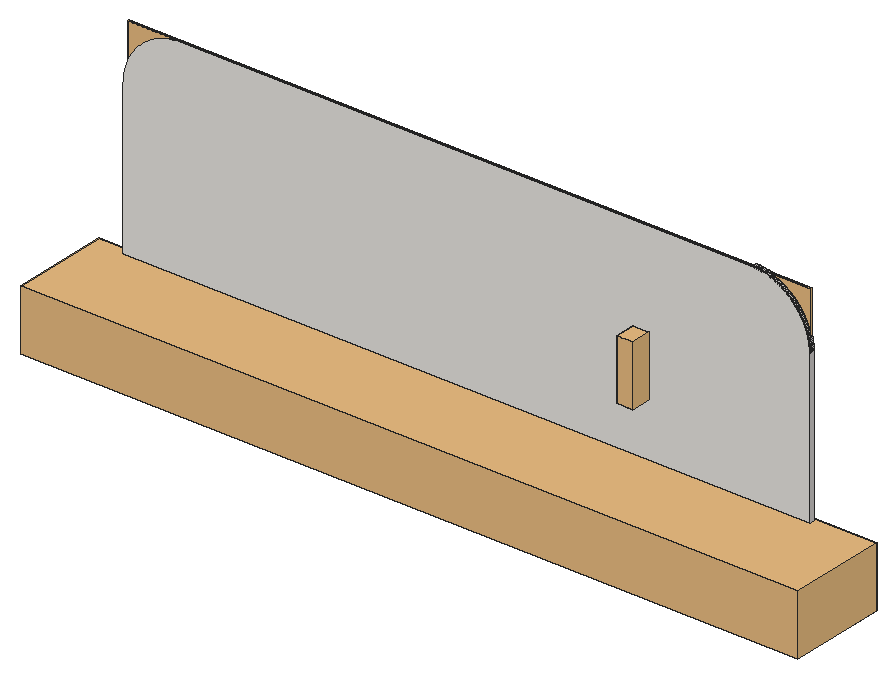
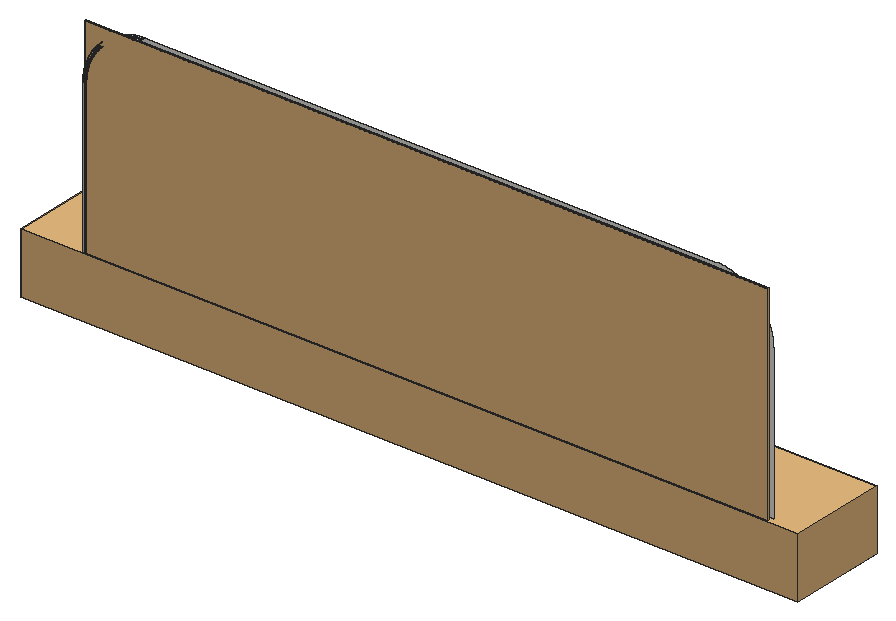
# SketchUp Ruby script. Lengths in inches.
U = 1.inch
M = Sketchup.active_model
def pt(a) = Geom::Point3d.new(a.map { |v| v * U })
def face(e, loops, mat)
  f = e.add_face(loops[0].map { |a| pt(a) })
  loops[1..].each { |l| e.add_face(l.map { |a| pt(a) }).erase! }
  f.material = f.back_material = mat if mat
  f
end
# faces: each face lists its corners as indices into pts; further lists are holes
def faces(e, pts, list, mat = nil) = list.each { |f| face(e, (f[0].is_a?(Array) ? f : [f]).map { |l| l.map { |i| pts[i] } }, mat) }
# xy, xz, yz: faces in a plane at the given z, y or x. An outline is a flat list of corners, or four numbers for a rectangle; further outlines are holes
def ring(l) = l.size == 4 ? [[l[0], l[1]], [l[2], l[1]], [l[2], l[3]], [l[0], l[3]]] : l.each_slice(2).to_a
def flat(e, list, mat, &to3) = list.each { |f| face(e, (f[0].is_a?(Array) ? f : [f]).map { |l| ring(l).map { |u, v| to3.(u, v) } }, mat) }
def xy(e, z, list, mat = nil) = flat(e, list, mat) { |x, y| [x, y, z] }
def xz(e, y, list, mat = nil) = flat(e, list, mat) { |x, z| [x, y, z] }
def yz(e, x, list, mat = nil) = flat(e, list, mat) { |y, z| [x, y, z] }
def lines(e, pts, list) = list.each { |a, b| e.add_line(pt(pts[a]), pt(pts[b])) }
# prism: a flat outline (further loops are holes) pulled along v
def prism(e, loops, v, mat = nil)
  f = face(e, loops, mat); d = Geom::Vector3d.new(v.map { |x| x * U })
  f.pushpull(f.normal.samedirection?(d) ? d.length : -d.length)
end
def box(e, o, s, mat = nil) = prism(e, [[o, [o[0] + s[0], o[1], o[2]], [o[0] + s[0], o[1] + s[1], o[2]], [o[0], o[1] + s[1], o[2]]]], [0, 0, s[2]], mat)
def at(x, y, z, deg = 0) = Geom::Transformation.translation(pt([x, y, z])) * Geom::Transformation.rotation(ORIGIN, Z_AXIS, deg.degrees)
def axes(o, x, y, z) = Geom::Transformation.new([*x, 0, *y, 0, *z, 0, *pt(o).to_a, 1])
def part(name) = M.definitions.add(name)
# library, detail: a bought-in or finely detailed component or shape, given as its bounding box
def library(name, o, s) = part(name).tap { |d| box(d.entities, o, s) }
def detail(e, o, s) = box(e.add_group.entities, o, s)
def put(e, d, t, mat = nil) = e.add_instance(d, t).tap { |i| i.material = mat if mat }
def group(e, t, mat = nil) = e.add_group.tap { |g| g.transformation = t; g.material = mat if mat }.entities
root = M.entities
M.materials.add("Wall Light").color = [248, 221, 148]
M.materials.add("[Carrera Marble]").color = [233, 230, 225]
M.materials.add("[Stone Vein Gray]").color = [206, 202, 201]
M.materials.add("[Wood Cherry Original]").color = [91, 49, 20]
c1 = library("Group\#3",[0,0,0],[135.3,0.25,52.8])
c2 = library("Group\#6",[-6,0,0],[154,19.5,12])
c3 = library("WALL LIGHT 69",[4.19,4.05,-8.78],[4.61,5.7,17.13])
xy(root,0.35,[[307.85,83.25,308.15,83.5]])
xy(root,53.48,[[297.6,82.5,297.75,83.5]],"[Stone Vein Gray]")
xy(root,53.5,[[297,82.5,297.15,83.5],[297.15,82.5,297.3,83.5]],"[Stone Vein Gray]")
xz(root,82.5,[[172.5,0,308.5,0,308.5,42.3,308.48,42.6,308.48,42.75,308.46,42.9,308.45,43.05,308.4375,43.2,308.42,43.35,308.36,43.8,308.33,43.95,308.31,44.1,308.28,44.24,308.22,44.54,308.18,44.68,308.15,44.83,308.11,44.98,308.07,45.12,308.03,45.27,307.98,45.41,307.9375,45.55,307.89,45.7,307.74,46.12,307.68,46.26,307.57,46.54,307.51,46.68,307.44,46.81,307.38,46.95,307.3125,47.09,307.25,47.22,307.18,47.35,307.11,47.49,307.03,47.62,306.96,47.75,306.88,47.88,306.81,48.01,306.73,48.14,306.64,48.26,306.5625,48.39,306.48,48.51,306.39,48.64,306.21,48.88,306.125,49,306.03,49.12,305.9375,49.24,305.84,49.35,305.74,49.47,305.65,49.58,305.55,49.7,305.44,49.81,305.34,49.92,304.92,50.34,304.81,50.44,304.7,50.55,304.58,50.65,304.47,50.74,304.35,50.84,304.24,50.9375,304.12,51.03,304,51.125,303.88,51.21,303.64,51.39,303.51,51.48,303.39,51.5625,303.26,51.64,303.14,51.73,303.01,51.81,302.88,51.88,302.75,51.96,302.62,52.03,302.49,52.11,302.35,52.18,302.22,52.25,302.09,52.3125,301.95,52.38,301.81,52.44,301.68,52.51,301.54,52.57,301.26,52.68,301.12,52.74,300.7,52.89,300.55,52.9375,300.41,52.98,300.27,53.03,300.12,53.07,299.98,53.11,299.83,53.15,299.68,53.18,299.54,53.22,299.24,53.28,299.1,53.31,298.95,53.33,298.8,53.36,298.35,53.42,298.2,53.4375,298.05,53.45,297.9,53.46,297.75,53.48,297.6,53.48,297.3,53.5,183.7,53.5,183.4,53.48,183.25,53.48,183.1,53.46,182.95,53.45,182.8,53.4375,182.65,53.42,182.2,53.36,182.05,53.33,181.9,53.31,181.76,53.28,181.46,53.22,181.32,53.18,181.17,53.15,181.02,53.11,180.88,53.07,180.73,53.03,180.59,52.98,180.45,52.9375,180.3,52.89,179.88,52.74,179.74,52.68,179.46,52.57,179.32,52.51,179.19,52.44,179.05,52.38,178.91,52.3125,178.78,52.25,178.65,52.18,178.51,52.11,178.38,52.03,178.25,51.96,178.12,51.88,177.99,51.81,177.86,51.73,177.74,51.64,177.61,51.5625,177.49,51.48,177.36,51.39,177.12,51.21,177,51.125,176.88,51.03,176.76,50.9375,176.65,50.84,176.53,50.74,176.42,50.65,176.3,50.55,176.19,50.44,176.08,50.34,175.66,49.92,175.56,49.81,175.45,49.7,175.35,49.58,175.26,49.47,175.16,49.35,175.0625,49.24,174.97,49.12,174.875,49,174.79,48.88,174.61,48.64,174.52,48.51,174.4375,48.39,174.36,48.26,174.27,48.14,174.19,48.01,174.12,47.88,174.04,47.75,173.97,47.62,173.89,47.49,173.82,47.35,173.75,47.22,173.6875,47.09,173.62,46.95,173.56,46.81,173.49,46.68,173.43,46.54,173.32,46.26,173.26,46.12,173.11,45.7,173.0625,45.55,173.02,45.41,172.97,45.27,172.93,45.12,172.89,44.98,172.85,44.83,172.82,44.68,172.78,44.54,172.72,44.24,172.69,44.1,172.67,43.95,172.64,43.8,172.58,43.35,172.5625,43.2,172.55,43.05,172.54,42.9,172.52,42.75,172.52,42.6,172.5,42.3]],"[Carrera Marble]")
xz(root,83.25,[[307.85,0,308.15,0.35],[172.85,0.35,172.85,42.29,172.86,42.4375,172.87,42.58,172.875,42.73,172.88,42.875,172.9,43.02,172.91,43.17,172.93,43.3125,172.95,43.46,172.99,43.74,173.01,43.89,173.04,44.03,173.0625,44.18,173.09,44.32,173.16,44.6,173.19,44.74,173.23,44.89,173.35,45.31,173.4,45.45,173.44,45.58,173.59,46,173.64,46.13,173.7,46.27,173.76,46.4,173.8125,46.54,174,46.93,174.07,47.0625,174.13,47.19,174.27,47.45,174.34,47.57,174.42,47.7,174.49,47.83,174.73,48.19,174.8125,48.32,174.89,48.44,174.98,48.55,175.07,48.67,175.15,48.79,175.24,48.9,175.33,49.02,175.43,49.13,175.52,49.24,175.62,49.35,175.71,49.46,175.8125,49.57,175.91,49.68,176.01,49.78,176.12,49.88,176.22,49.99,176.32,50.09,176.43,50.1875,176.54,50.29,176.65,50.38,176.76,50.48,176.87,50.57,176.98,50.67,177.1,50.76,177.21,50.85,177.33,50.93,177.45,51.02,177.56,51.11,177.68,51.1875,177.81,51.27,178.17,51.51,178.3,51.58,178.42,51.66,178.81,51.87,178.9375,51.93,179.07,52,179.46,52.1875,179.6,52.24,179.73,52.3,179.87,52.36,180,52.41,180.42,52.56,180.55,52.6,180.69,52.65,181.11,52.77,181.26,52.81,181.4,52.84,181.68,52.91,181.82,52.9375,181.97,52.96,182.11,52.99,182.26,53.01,182.54,53.05,182.6875,53.07,182.83,53.09,182.98,53.1,183.125,53.12,183.27,53.125,183.42,53.13,183.5625,53.14,183.71,53.15,297.29,53.15,297.4375,53.14,297.58,53.13,297.73,53.125,297.875,53.12,298.02,53.1,298.17,53.09,298.3125,53.07,298.46,53.05,298.74,53.01,298.89,52.99,299.03,52.96,299.18,52.9375,299.32,52.91,299.6,52.84,299.74,52.81,299.89,52.77,300.31,52.65,300.45,52.6,300.58,52.56,301,52.41,301.13,52.36,301.27,52.3,301.4,52.24,301.54,52.1875,301.93,52,302.0625,51.93,302.19,51.87,302.58,51.66,302.7,51.58,302.83,51.51,303.19,51.27,303.32,51.1875,303.44,51.11,303.55,51.02,303.67,50.93,303.79,50.85,303.9,50.76,304.02,50.67,304.13,50.57,304.24,50.48,304.35,50.38,304.46,50.29,304.57,50.1875,304.68,50.09,304.78,49.99,304.88,49.88,304.99,49.78,305.09,49.68,305.1875,49.57,305.29,49.46,305.38,49.35,305.48,49.24,305.57,49.13,305.67,49.02,305.76,48.9,305.85,48.79,305.93,48.67,306.02,48.55,306.11,48.44,306.1875,48.32,306.27,48.19,306.51,47.83,306.58,47.7,306.66,47.58,306.87,47.19,306.93,47.0625,307,46.93,307.1875,46.54,307.24,46.4,307.3,46.27,307.36,46.13,307.41,46,307.56,45.58,307.6,45.45,307.65,45.31,307.77,44.89,307.81,44.74,307.84,44.6,307.91,44.32,307.9375,44.18,307.96,44.03,307.99,43.89,308.01,43.74,308.05,43.46,308.07,43.3125,308.09,43.17,308.1,43.02,308.12,42.875,308.125,42.73,308.13,42.58,308.14,42.4375,308.15,42.29,308.15,0.35,307.85,0.35,307.85,42.28,307.84,42.43,307.84,42.57,307.82,42.85,307.8,42.99,307.79,43.13,307.77,43.28,307.76,43.42,307.72,43.7,307.69,43.84,307.67,43.98,307.61,44.26,307.58,44.39,307.52,44.67,307.44,44.95,307.4,45.08,307.36,45.22,307.32,45.35,307.27,45.49,307.23,45.62,307.18,45.76,307.08,46.02,307.02,46.15,306.97,46.28,306.67,46.93,306.6,47.05,306.54,47.18,306.47,47.3,306.4,47.43,306.32,47.55,306.18,47.79,305.94,48.15,305.86,48.26,305.78,48.38,305.69,48.49,305.61,48.61,305.43,48.83,305.34,48.9375,305.25,49.05,305.16,49.15,305.0625,49.26,304.97,49.36,304.87,49.47,304.47,49.87,304.36,49.97,304.26,50.0625,304.15,50.16,304.05,50.25,303.9375,50.34,303.83,50.43,303.61,50.61,303.49,50.69,303.38,50.78,303.26,50.86,303.15,50.94,302.79,51.18,302.55,51.32,302.42,51.4,302.18,51.54,302.05,51.6,301.93,51.67,301.28,51.97,301.15,52.02,301.02,52.08,300.76,52.18,300.62,52.23,300.49,52.27,300.35,52.32,300.22,52.36,300.08,52.4,299.95,52.44,299.67,52.52,299.39,52.58,299.26,52.61,298.98,52.67,298.84,52.69,298.7,52.72,298.42,52.76,298.28,52.77,298.13,52.79,297.99,52.8,297.85,52.82,297.57,52.84,297.43,52.84,297.28,52.85,183.72,52.85,183.57,52.84,183.43,52.84,183.15,52.82,183.01,52.8,182.87,52.79,182.72,52.77,182.58,52.76,182.3,52.72,182.16,52.69,182.02,52.67,181.74,52.61,181.61,52.58,181.33,52.52,181.05,52.44,180.92,52.4,180.78,52.36,180.65,52.32,180.51,52.27,180.38,52.23,180.24,52.18,179.98,52.08,179.85,52.02,179.72,51.97,179.07,51.67,178.95,51.6,178.82,51.54,178.58,51.4,178.45,51.32,178.21,51.18,177.85,50.94,177.74,50.86,177.62,50.78,177.51,50.69,177.39,50.61,177.17,50.43,177.0625,50.34,176.95,50.25,176.85,50.16,176.74,50.0625,176.64,49.97,176.53,49.87,176.13,49.47,176.03,49.36,175.9375,49.26,175.84,49.15,175.75,49.05,175.66,48.9375,175.57,48.83,175.39,48.61,175.31,48.49,175.22,48.38,175.14,48.26,175.06,48.15,174.82,47.79,174.68,47.55,174.6,47.42,174.46,47.18,174.4,47.05,174.33,46.93,174.03,46.28,173.98,46.15,173.92,46.02,173.82,45.76,173.77,45.62,173.73,45.49,173.68,45.35,173.64,45.22,173.6,45.08,173.56,44.95,173.48,44.67,173.42,44.39,173.39,44.26,173.33,43.98,173.31,43.84,173.28,43.7,173.24,43.42,173.23,43.28,173.21,43.13,173.2,42.99,173.18,42.85,173.16,42.57,173.16,42.43,173.15,42.28,173.15,0.35]])
yz(root,307.84,[[83.25,42.43,83.5,42.57]])
yz(root,307.85,[[83.25,0,83.5,0.35],[83.25,0.35,83.5,42],[83.25,42,83.5,42.14],[83.25,42.14,83.5,42.28]])
yz(root,308.15,[[83.25,0,83.5,0.35],[83.25,0.35,83.5,42],[83.25,42,83.5,42.15],[83.25,42.15,83.5,42.29]])
yz(root,308.48,[[82.5,42.6,83.5,42.75]],"[Stone Vein Gray]")
yz(root,308.5,[[82.5,0,83.5,42],[82.5,42,83.5,42.15],[82.5,42.15,83.5,42.3]],"[Stone Vein Gray]")
p = [[308.5,83.5,42.3],[308.49,83.5,42.45],[308.49,82.5,42.45],[308.5,82.5,42.3],[307.85,83.5,42.28],[307.84,83.5,42.43],
  [307.84,83.25,42.43],[307.85,83.25,42.28],[308.14,83.5,42.4375],[308.15,83.5,42.29],[308.15,83.25,42.29],[308.14,83.25,42.4375],
  [308.13,83.5,42.58],[308.13,83.25,42.58],[308.48,83.5,42.6],[308.48,82.5,42.6],[307.84,83.5,42.57],[307.83,83.5,42.71],
  [307.83,83.25,42.71],[307.84,83.25,42.57],[308.125,83.5,42.73],[308.125,83.25,42.73],[307.82,83.5,42.85],[307.82,83.25,42.85],
  [308.12,83.5,42.875],[308.12,83.25,42.875],[308.48,83.5,42.75],[308.46,83.5,42.9],[308.46,82.5,42.9],[308.48,82.5,42.75],
  [308.45,83.5,43.05],[308.45,82.5,43.05],[307.8,83.5,42.99],[307.8,83.25,42.99],[308.1,83.5,43.02],[308.1,83.25,43.02],
  [307.79,83.5,43.13],[307.79,83.25,43.13],[308.09,83.5,43.17],[308.09,83.25,43.17],[308.4375,83.5,43.2],[308.4375,82.5,43.2],
  [307.77,83.5,43.28],[307.77,83.25,43.28],[308.42,83.5,43.35],[308.42,82.5,43.35],[308.07,83.5,43.3125],[308.07,83.25,43.3125],
  [307.76,83.5,43.42],[307.76,83.25,43.42],[308.05,83.5,43.46],[308.05,83.25,43.46],[308.4,83.5,43.5],[308.4,82.5,43.5],
  [307.74,83.5,43.56],[307.74,83.25,43.56],[308.38,83.5,43.65],[308.38,82.5,43.65],[308.03,83.5,43.6],[308.03,83.25,43.6],
  [307.72,83.5,43.7],[307.72,83.25,43.7],[308.01,83.5,43.74],[308.01,83.25,43.74],[308.36,83.5,43.8],[308.36,82.5,43.8],
  [307.69,83.5,43.84],[307.69,83.25,43.84],[307.99,83.5,43.89],[307.99,83.25,43.89],[308.33,83.5,43.95],[308.33,82.5,43.95],
  [307.67,83.5,43.98],[307.67,83.25,43.98],[308.31,83.5,44.1],[308.31,82.5,44.1],[307.96,83.5,44.03],[307.96,83.25,44.03],
  [307.64,83.5,44.12],[307.64,83.25,44.12],[307.9375,83.5,44.18],[307.9375,83.25,44.18],[308.28,83.5,44.24],[308.28,82.5,44.24],
  [307.61,83.5,44.26],[307.61,83.25,44.26],[308.25,83.5,44.39],[308.25,82.5,44.39],[307.91,83.5,44.32],[307.91,83.25,44.32],
  [307.58,83.5,44.39],[307.58,83.25,44.39],[307.875,83.5,44.46],[307.875,83.25,44.46],[308.22,83.5,44.54],[308.22,82.5,44.54],
  [307.55,83.5,44.53],[307.55,83.25,44.53],[308.18,83.5,44.68],[308.18,82.5,44.68],[307.52,83.5,44.67],[307.52,83.25,44.67],
  [307.84,83.5,44.6],[307.84,83.25,44.6],[307.81,83.5,44.74],[307.81,83.25,44.74],[308.15,83.5,44.83],[308.15,82.5,44.83],
  [307.48,83.5,44.81],[307.48,83.25,44.81],[307.77,83.5,44.89],[307.77,83.25,44.89],[308.11,83.5,44.98],[308.11,82.5,44.98],
  [307.44,83.5,44.95],[307.44,83.25,44.95],[307.4,83.5,45.08],[307.4,83.25,45.08],[307.73,83.5,45.03],[307.73,83.25,45.03],
  [308.07,83.5,45.12],[308.07,82.5,45.12],[307.69,83.5,45.17],[307.69,83.25,45.17],[308.03,83.5,45.27],[308.03,82.5,45.27],
  [307.36,83.5,45.22],[307.36,83.25,45.22],[307.32,83.5,45.35],[307.32,83.25,45.35],[307.65,83.5,45.31],[307.65,83.25,45.31],
  [307.98,83.5,45.41],[307.98,82.5,45.41],[307.6,83.5,45.45],[307.6,83.25,45.45],[307.9375,83.5,45.55],[307.9375,82.5,45.55],
  [307.27,83.5,45.49],[307.27,83.25,45.49],[307.56,83.5,45.58],[307.56,83.25,45.58],[307.23,83.5,45.62],[307.23,83.25,45.62],
  [307.89,83.5,45.7],[307.89,82.5,45.7],[307.18,83.5,45.76],[307.18,83.25,45.76],[307.51,83.5,45.72],[307.51,83.25,45.72],
  [307.84,83.5,45.84],[307.84,82.5,45.84],[307.46,83.5,45.86],[307.46,83.25,45.86],[307.79,83.5,45.98],[307.79,82.5,45.98],
  [307.13,83.5,45.89],[307.13,83.25,45.89],[307.08,83.5,46.02],[307.08,83.25,46.02],[307.41,83.5,46],[307.41,83.25,46],
  [307.74,83.5,46.12],[307.74,82.5,46.12],[307.02,83.5,46.15],[307.02,83.25,46.15],[307.36,83.5,46.13],[307.36,83.25,46.13],
  [307.68,83.5,46.26],[307.68,82.5,46.26],[307.3,83.5,46.27],[307.3,83.25,46.27],[306.97,83.5,46.28],[306.97,83.25,46.28],
  [307.625,83.5,46.4],[307.625,82.5,46.4],[306.91,83.5,46.41],[306.91,83.25,46.41],[307.24,83.5,46.4],[307.24,83.25,46.4],
  [307.57,83.5,46.54],[307.57,82.5,46.54],[306.85,83.5,46.54],[306.85,83.25,46.54],[307.1875,83.5,46.54],[307.1875,83.25,46.54],
  [307.51,83.5,46.68],[307.51,82.5,46.68],[306.79,83.5,46.67],[306.79,83.25,46.67],[307.125,83.5,46.67],[307.125,83.25,46.67],
  [307.44,83.5,46.81],[307.44,82.5,46.81],[306.73,83.5,46.8],[306.73,83.25,46.8],[307.0625,83.5,46.8],[307.0625,83.25,46.8],
  [307.38,83.5,46.95],[307.38,82.5,46.95],[306.67,83.5,46.93],[306.67,83.25,46.93],[307,83.5,46.93],[307,83.25,46.93],
  [306.6,83.5,47.05],[306.6,83.25,47.05],[306.93,83.5,47.0625],[306.93,83.25,47.0625],[307.3125,83.5,47.09],[307.3125,82.5,47.09],
  [307.25,83.5,47.22],[307.25,82.5,47.22],[306.54,83.5,47.18],[306.54,83.25,47.18],[306.87,83.5,47.19],[306.87,83.25,47.19],
  [307.18,83.5,47.35],[307.18,82.5,47.35],[306.47,83.5,47.3],[306.47,83.25,47.3],[306.8,83.5,47.32],[306.8,83.25,47.32],
  [306.4,83.5,47.43],[306.4,83.25,47.43],[306.73,83.5,47.45],[306.73,83.25,47.45],[307.11,83.5,47.49],[307.11,82.5,47.49],
  [306.32,83.5,47.55],[306.32,83.25,47.55],[306.66,83.5,47.58],[306.66,83.25,47.58],[307.03,83.5,47.62],[307.03,82.5,47.62],
  [306.25,83.5,47.67],[306.25,83.25,47.67],[306.96,83.5,47.75],[306.96,82.5,47.75],[306.58,83.5,47.7],[306.58,83.25,47.7],
  [306.18,83.5,47.79],[306.18,83.25,47.79],[306.51,83.5,47.83],[306.51,83.25,47.83],[306.88,83.5,47.88],[306.88,82.5,47.88],
  [306.1,83.5,47.91],[306.1,83.25,47.91],[306.43,83.5,47.95],[306.43,83.25,47.95],[306.81,83.5,48.01],[306.81,82.5,48.01],
  [306.02,83.5,48.03],[306.02,83.25,48.03],[306.35,83.5,48.07],[306.35,83.25,48.07],[306.73,83.5,48.14],[306.73,82.5,48.14],
  [305.94,83.5,48.15],[305.94,83.25,48.15],[306.64,83.5,48.26],[306.64,82.5,48.26],[305.86,83.5,48.26],[305.86,83.25,48.26],
  [306.27,83.5,48.19],[306.27,83.25,48.19],[306.1875,83.5,48.32],[306.1875,83.25,48.32],[306.5625,83.5,48.39],[306.5625,82.5,48.39],
  [305.78,83.5,48.38],[305.78,83.25,48.38],[306.11,83.5,48.44],[306.11,83.25,48.44],[306.48,83.5,48.51],[306.48,82.5,48.51],
  [305.69,83.5,48.49],[305.69,83.25,48.49],[306.02,83.5,48.55],[306.02,83.25,48.55],[306.39,83.5,48.64],[306.39,82.5,48.64],
  [305.61,83.5,48.61],[305.61,83.25,48.61],[306.3,83.5,48.76],[306.3,82.5,48.76],[305.52,83.5,48.72],[305.52,83.25,48.72],
  [305.93,83.5,48.67],[305.93,83.25,48.67],[305.43,83.5,48.83],[305.43,83.25,48.83],[305.85,83.5,48.79],[305.85,83.25,48.79],
  [306.21,83.5,48.88],[306.21,82.5,48.88],[305.34,83.5,48.9375],[305.34,83.25,48.9375],[305.76,83.5,48.9],[305.76,83.25,48.9],
  [306.125,83.5,49],[306.125,82.5,49],[305.25,83.5,49.05],[305.25,83.25,49.05],[305.67,83.5,49.02],[305.67,83.25,49.02],
  [306.03,83.5,49.12],[306.03,82.5,49.12],[305.16,83.5,49.15],[305.16,83.25,49.15],[305.57,83.5,49.13],[305.57,83.25,49.13],
  [305.9375,83.5,49.24],[305.9375,82.5,49.24],[305.48,83.5,49.24],[305.48,83.25,49.24],[305.84,83.5,49.35],[305.84,82.5,49.35],
  [305.0625,83.5,49.26],[305.0625,83.25,49.26],[305.38,83.5,49.35],[305.38,83.25,49.35],[304.97,83.5,49.36],[304.97,83.25,49.36],
  [305.74,83.5,49.47],[305.74,82.5,49.47],[304.87,83.5,49.47],[304.87,83.25,49.47],[305.29,83.5,49.46],[305.29,83.25,49.46],
  [305.65,83.5,49.58],[305.65,82.5,49.58],[304.77,83.5,49.57],[304.77,83.25,49.57],[305.1875,83.5,49.57],[305.1875,83.25,49.57],
  [305.55,83.5,49.7],[305.55,82.5,49.7],[304.67,83.5,49.67],[304.67,83.25,49.67],[305.09,83.5,49.68],[305.09,83.25,49.68],
  [305.44,83.5,49.81],[305.44,82.5,49.81],[304.57,83.5,49.77],[304.57,83.25,49.77],[304.99,83.5,49.78],[304.99,83.25,49.78],
  [305.34,83.5,49.92],[305.34,82.5,49.92],[305.24,83.5,50.02],[305.24,82.5,50.02],[305.13,83.5,50.13],[305.13,82.5,50.13],
  [305.02,83.5,50.24],[305.02,82.5,50.24],[304.92,83.5,50.34],[304.92,82.5,50.34],[304.81,83.5,50.44],[304.81,82.5,50.44],
  [304.7,83.5,50.55],[304.7,82.5,50.55],[304.58,83.5,50.65],[304.58,82.5,50.65],[304.47,83.5,50.74],[304.47,82.5,50.74],
  [304.35,83.5,50.84],[304.35,82.5,50.84],[304.24,83.5,50.9375],[304.24,82.5,50.9375],[304.12,83.5,51.03],[304.12,82.5,51.03],
  [304,83.5,51.125],[304,82.5,51.125],[303.88,83.5,51.21],[303.88,82.5,51.21],[303.76,83.5,51.3],[303.76,82.5,51.3],
  [303.64,83.5,51.39],[303.64,82.5,51.39],[303.51,83.5,51.48],[303.51,82.5,51.48],[303.39,83.5,51.5625],[303.39,82.5,51.5625],
  [303.26,83.5,51.64],[303.14,83.5,51.73],[303.14,82.5,51.73],[303.26,82.5,51.64],[303.01,83.5,51.81],[303.01,82.5,51.81],
  [302.88,83.5,51.88],[302.88,82.5,51.88],[302.75,83.5,51.96],[302.75,82.5,51.96],[302.62,83.5,52.03],[302.49,83.5,52.11],
  [302.49,82.5,52.11],[302.62,82.5,52.03],[302.35,83.5,52.18],[302.35,82.5,52.18],[302.22,83.5,52.25],[302.09,83.5,52.3125],
  [302.09,82.5,52.3125],[302.22,82.5,52.25],[301.95,83.5,52.38],[301.95,82.5,52.38],[301.81,83.5,52.44],[301.68,83.5,52.51],
  [301.68,82.5,52.51],[301.81,82.5,52.44],[301.54,83.5,52.57],[301.54,82.5,52.57],[301.4,83.5,52.625],[301.26,83.5,52.68],
  [301.26,82.5,52.68],[301.4,82.5,52.625],[301.12,83.5,52.74],[300.98,83.5,52.79],[300.98,82.5,52.79],[301.12,82.5,52.74],
  [300.84,83.5,52.84],[300.7,83.5,52.89],[300.7,82.5,52.89],[300.84,82.5,52.84],[300.55,83.5,52.9375],[300.41,83.5,52.98],
  [300.41,82.5,52.98],[300.55,82.5,52.9375],[300.27,83.5,53.03],[300.12,83.5,53.07],[300.12,82.5,53.07],[300.27,82.5,53.03],
  [299.83,83.5,53.15],[299.68,83.5,53.18],[299.68,82.5,53.18],[299.83,82.5,53.15],[299.98,83.5,53.11],[299.98,82.5,53.11],
  [299.39,83.5,53.25],[299.24,83.5,53.28],[299.24,82.5,53.28],[299.39,82.5,53.25],[299.54,83.5,53.22],[299.54,82.5,53.22],
  [298.95,83.5,53.33],[298.8,83.5,53.36],[298.8,82.5,53.36],[298.95,82.5,53.33],[299.1,83.5,53.31],[299.1,82.5,53.31],
  [298.2,83.5,53.4375],[298.05,83.5,53.45],[298.05,82.5,53.45],[298.2,82.5,53.4375],[298.35,83.5,53.42],[298.35,82.5,53.42],
  [298.5,83.5,53.4],[298.5,82.5,53.4],[298.65,83.5,53.38],[298.65,82.5,53.38],[297.45,83.5,53.49],[297.3,83.5,53.5],
  [297.3,82.5,53.5],[297.45,82.5,53.49],[297.6,83.5,53.48],[297.6,82.5,53.48],[297.9,83.5,53.46],[297.75,83.5,53.48],
  [297.75,82.5,53.48],[297.9,82.5,53.46]]
faces(root,p,[[0,1,2,3],[1,14,15,2],[26,27,28,29],[27,30,31,28],[30,40,41,31],[40,44,45,41],[44,52,53,45],[52,56,57,53],
  [56,64,65,57],[64,70,71,65],[70,74,75,71],[74,82,83,75],[82,86,87,83],[86,94,95,87],[94,98,99,95],[98,106,107,99],
  [106,112,113,107],[112,120,121,113],[120,124,125,121],[124,132,133,125],[132,136,137,133],[136,144,145,137],[144,150,151,145],[150,154,155,151],
  [154,162,163,155],[162,168,169,163],[168,174,175,169],[174,180,181,175],[180,186,187,181],[186,192,193,187],[192,198,199,193],[198,208,209,199],
  [208,210,211,209],[210,216,217,211],[216,226,227,217],[226,232,233,227],[232,236,237,233],[236,244,245,237],[244,250,251,245],[250,256,257,251],
  [256,260,261,257],[260,268,269,261],[268,274,275,269],[274,280,281,275],[280,284,285,281],[284,294,295,285],[294,300,301,295],[300,306,307,301],
  [306,312,313,307],[312,316,317,313],[316,324,325,317],[324,330,331,325],[330,336,337,331],[336,342,343,337],[342,348,349,343],[348,350,351,349],
  [350,352,353,351],[352,354,355,353],[354,356,357,355],[356,358,359,357],[358,360,361,359],[360,362,363,361],[362,364,365,363],[364,366,367,365],
  [366,368,369,367],[368,370,371,369],[370,372,373,371],[372,374,375,373],[374,376,377,375],[376,378,379,377],[378,380,381,379],[380,382,383,381],
  [384,385,386,387],[382,384,387,383],[385,388,389,386],[388,390,391,389],[390,392,393,391],[394,395,396,397],[392,394,397,393],[395,398,399,396],
  [400,401,402,403],[398,400,403,399],[401,404,405,402],[406,407,408,409],[404,406,409,405],[407,410,411,408],[412,413,414,415],[410,412,415,411],
  [416,417,418,419],[413,416,419,414],[420,421,422,423],[417,420,423,418],[424,425,426,427],[421,424,427,422],[428,429,430,431],[425,428,431,426],
  [432,433,434,435],[436,432,435,437],[429,436,437,430],[438,439,440,441],[442,438,441,443],[433,442,443,434],[444,445,446,447],[448,444,447,449],
  [439,448,449,440],[450,451,452,453],[454,450,453,455],[456,454,455,457],[458,456,457,459],[445,458,459,446],[460,461,462,463],[464,460,463,465],
  [466,467,468,469],[451,466,469,452]],"[Stone Vein Gray]")
faces(root,p,[[4,5,6,7],[8,9,10,11],[12,8,11,13],[16,17,18,19],[20,12,13,21],[17,22,23,18],[24,20,21,25],[22,32,33,23],
  [34,24,25,35],[32,36,37,33],[38,34,35,39],[36,42,43,37],[46,38,39,47],[42,48,49,43],[50,46,47,51],[48,54,55,49],
  [58,50,51,59],[54,60,61,55],[62,58,59,63],[60,66,67,61],[68,62,63,69],[66,72,73,67],[76,68,69,77],[72,78,79,73],
  [80,76,77,81],[78,84,85,79],[88,80,81,89],[84,90,91,85],[92,88,89,93],[90,96,97,91],[96,100,101,97],[102,92,93,103],
  [104,102,103,105],[100,108,109,101],[110,104,105,111],[108,114,115,109],[114,116,117,115],[118,110,111,119],[122,118,119,123],[116,126,127,117],
  [126,128,129,127],[130,122,123,131],[134,130,131,135],[128,138,139,129],[140,134,135,141],[138,142,143,139],[142,146,147,143],[148,140,141,149],
  [152,148,149,153],[146,156,157,147],[156,158,159,157],[160,152,153,161],[158,164,165,159],[166,160,161,167],[170,166,167,171],[164,172,173,165],
  [172,176,177,173],[178,170,171,179],[176,182,183,177],[184,178,179,185],[182,188,189,183],[190,184,185,191],[188,194,195,189],[196,190,191,197],
  [194,200,201,195],[202,196,197,203],[200,204,205,201],[206,202,203,207],[204,212,213,205],[214,206,207,215],[212,218,219,213],[220,214,215,221],
  [218,222,223,219],[224,220,221,225],[222,228,229,223],[230,224,225,231],[228,234,235,229],[238,230,231,239],[234,240,241,235],[242,238,239,243],
  [240,246,247,241],[248,242,243,249],[246,252,253,247],[254,248,249,255],[252,258,259,253],[258,262,263,259],[264,254,255,265],[266,264,265,267],
  [262,270,271,263],[272,266,267,273],[270,276,277,271],[278,272,273,279],[276,282,283,277],[282,286,287,283],[288,278,279,289],[286,290,291,287],
  [292,288,289,293],[290,296,297,291],[298,292,293,299],[296,302,303,297],[304,298,299,305],[302,308,309,303],[310,304,305,311],[314,310,311,315],
  [308,318,319,309],[320,314,315,321],[318,322,323,319],[322,326,327,323],[328,320,321,329],[326,332,333,327],[334,328,329,335],[332,338,339,333],
  [340,334,335,341],[338,344,345,339],[346,340,341,347]])
put(root,c1,at(172.85,83.25,0.35),"Wall Light")
put(root,c2,at(172.5,64.5,0),"[Wood Cherry Original]")
put(root,c3,axes([270.51,75.68,28.83],[0.7,0,0],[0,0.7,0],[0,0,0.7]))
